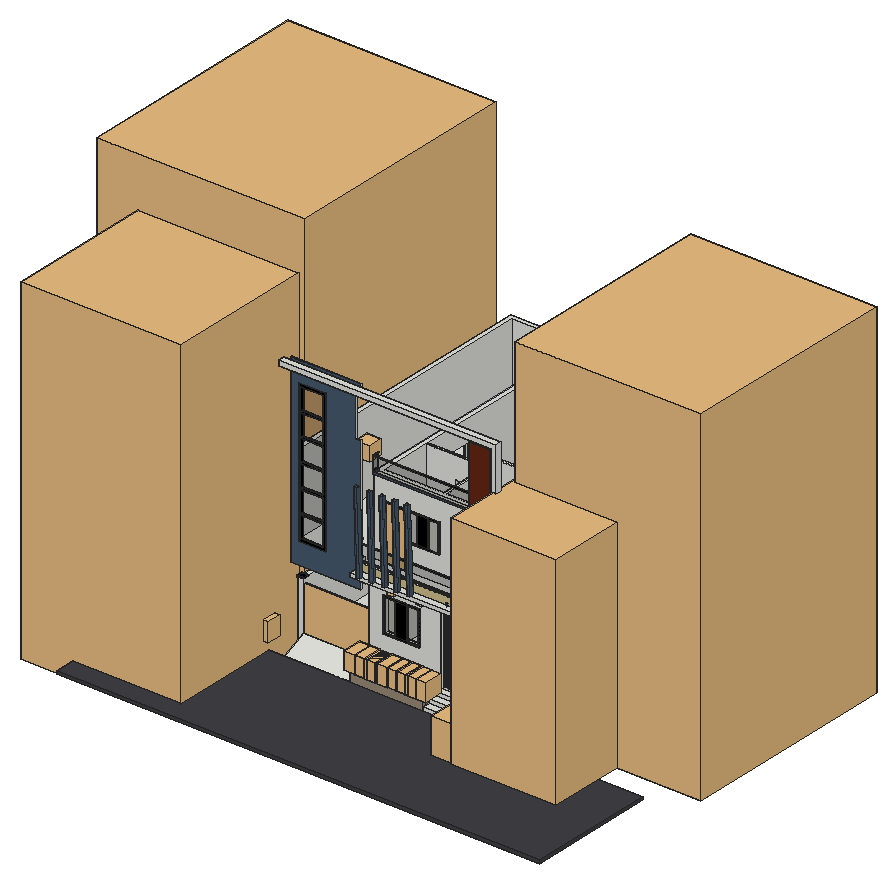
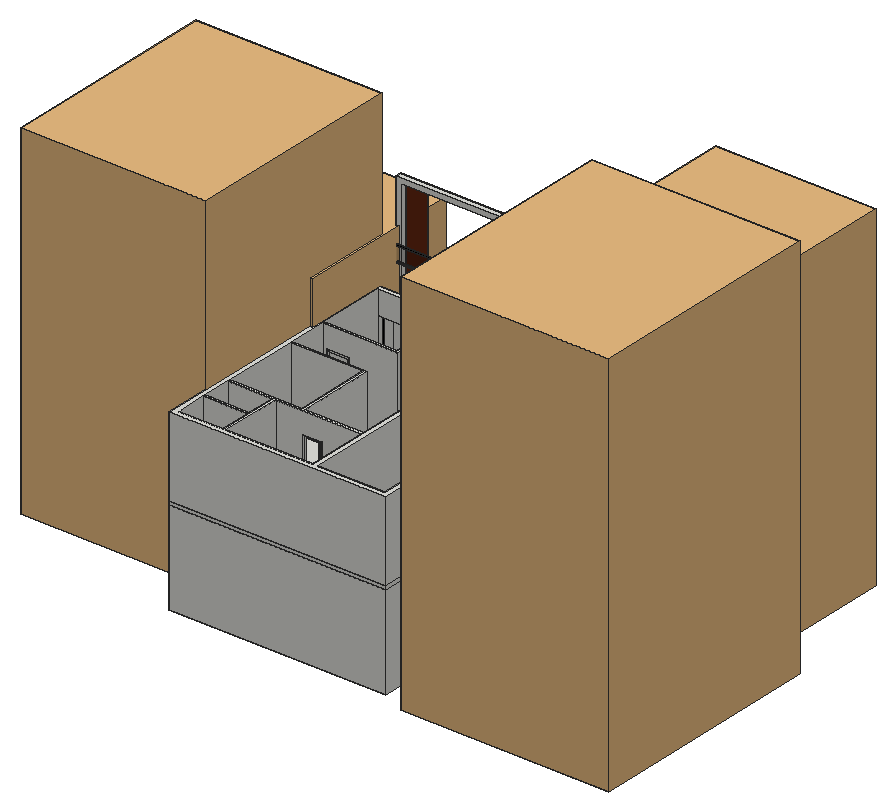
# SketchUp Ruby script. Lengths in inches.
U = 1.inch
M = Sketchup.active_model
def pt(a) = Geom::Point3d.new(a.map { |v| v * U })
def face(e, loops, mat)
  f = e.add_face(loops[0].map { |a| pt(a) })
  loops[1..].each { |l| e.add_face(l.map { |a| pt(a) }).erase! }
  f.material = f.back_material = mat if mat
  f
end
# faces: each face lists its corners as indices into pts; further lists are holes
def faces(e, pts, list, mat = nil) = list.each { |f| face(e, (f[0].is_a?(Array) ? f : [f]).map { |l| l.map { |i| pts[i] } }, mat) }
# xy, xz, yz: faces in a plane at the given z, y or x. An outline is a flat list of corners, or four numbers for a rectangle; further outlines are holes
def ring(l) = l.size == 4 ? [[l[0], l[1]], [l[2], l[1]], [l[2], l[3]], [l[0], l[3]]] : l.each_slice(2).to_a
def flat(e, list, mat, &to3) = list.each { |f| face(e, (f[0].is_a?(Array) ? f : [f]).map { |l| ring(l).map { |u, v| to3.(u, v) } }, mat) }
def xy(e, z, list, mat = nil) = flat(e, list, mat) { |x, y| [x, y, z] }
def xz(e, y, list, mat = nil) = flat(e, list, mat) { |x, z| [x, y, z] }
def yz(e, x, list, mat = nil) = flat(e, list, mat) { |y, z| [x, y, z] }
def lines(e, pts, list) = list.each { |a, b| e.add_line(pt(pts[a]), pt(pts[b])) }
# prism: a flat outline (further loops are holes) pulled along v
def prism(e, loops, v, mat = nil)
  f = face(e, loops, mat); d = Geom::Vector3d.new(v.map { |x| x * U })
  f.pushpull(f.normal.samedirection?(d) ? d.length : -d.length)
end
def box(e, o, s, mat = nil) = prism(e, [[o, [o[0] + s[0], o[1], o[2]], [o[0] + s[0], o[1] + s[1], o[2]], [o[0], o[1] + s[1], o[2]]]], [0, 0, s[2]], mat)
def at(x, y, z, deg = 0) = Geom::Transformation.translation(pt([x, y, z])) * Geom::Transformation.rotation(ORIGIN, Z_AXIS, deg.degrees)
def axes(o, x, y, z) = Geom::Transformation.new([*x, 0, *y, 0, *z, 0, *pt(o).to_a, 1])
def part(name) = M.definitions.add(name)
# library, detail: a bought-in or finely detailed component or shape, given as its bounding box
def library(name, o, s) = part(name).tap { |d| box(d.entities, o, s) }
def detail(e, o, s) = box(e.add_group.entities, o, s)
def put(e, d, t, mat = nil) = e.add_instance(d, t).tap { |i| i.material = mat if mat }
def group(e, t, mat = nil) = e.add_group.tap { |g| g.transformation = t; g.material = mat if mat }.entities
root = M.entities
M.materials.add("Asphalt Black 15-01 100cm").color = [65, 65, 69]
M.materials.add("GLass").color = [0, 0, 0]
M.materials["GLass"].alpha = 0.1
M.materials.add("Wall Paint Bumpy 01 Ochre 100cm").color = [152, 138, 118]
M.materials.add("Wall Paint Fine Grain 01 Yellow 100cm").color = [207, 190, 139]
M.materials.add("Wall Paint Simple Reflective").color = [70, 89, 109]
M.materials.add("Wood Dark 02 100cm").color = [99, 39, 19]
M.materials.add("metal").color = [0, 0, 0]
c1 = library("Tilia x europaea Pallida 007",[-304.07,-262.58,-28.16],[578.03,543.87,878])
c2 = part("Group\#50")
prism(c2.entities,[[[0,0,1.08],[0,0.04,0.8],[0,0.14,0.54],[0,0.32,0.32],[0,0.54,0.14],[0,0.8,0.04],[0,1.08,0],[0,1.36,0.04],[0,1.62,0.14],[0,1.84,0.3125],[0,1.84,1.84],[0,1.62,2.01],[0,1.36,2.12],[0,1.08,2.16],[0,0.8,2.12],[0,0.54,2.01],[0,0.32,1.84],[0,0.14,1.62],[0,0.04,1.36]]],[-101.4375,0,0])
c3 = library("Car 033",[-43.24,-98.19,-1.29],[86.48,201.64,57.79])
c4 = library("Schefflera arboricola 001",[-25.43,-22.82,-0.1],[47.76,45.73,64.24])
c5 = library("gate 134k",[0,0.67,0],[137.24,3.27,101.3])
c6 = library("Dome Light",[-12,-12,0],[24,24,12])
c7 = library("Omni Light\#2",[-12,-12,-12],[24,24,24])
c8 = library("Spot Light\#20",[-5.1,-5.1,-11.05],[10.2,10.2,11.05])
c9 = library("Spot Light\#21",[-5.1,-5.1,-11.05],[10.2,10.2,11.05])
c10 = library("Spot Light\#22",[-5.1,-5.1,-11.05],[10.2,10.2,11.05])
c11 = library("Spot Light\#23",[-5.1,-5.1,-11.05],[10.2,10.2,11.05])
c12 = library("Spot Light\#25",[-5.1,-5.1,-11.05],[10.2,10.2,11.05])
c13 = library("Spot Light\#24",[-5.1,-5.1,-11.05],[10.2,10.2,11.05])
c14 = library("Door 01",[-21.26,-2.6,0],[42.52,9.29,84.25])
c15 = library("Omni Light",[-12,-12,-12],[24,24,24])
put(root,c1,axes([25.28,470.38,-7.51],[0.59815,0,0],[0,0.73,0],[0,0,0.7332]))
put(root,c1,axes([52.75,315.37,-10.19],[0.4615,0,0],[0,1.07,0],[0,0,0.63803]))
g1 = group(root,at(197.75,0,0),"Asphalt Black 15-01 100cm")
box(g1,[-197.75,0,-5],[801.4375,215.125,5],"Asphalt Black 15-01 100cm")
g2 = group(root,at(436.25,190.68,5.33))
box(g2,[0,23.79,-6],[110.4375,39.41,6])
g3 = group(root,at(206.75,214.47,17.33))
prism(g3,[[[0,0,-17.33],[0,39.41,0],[0,39.41,-17.33]]],[108,0,0])
g4 = group(root,at(196.75,251.125,0))
g5 = group(g4,at(143.5,2.76,63.56))
xy(g5,0,[[0,-1.84,60,0]],"metal")
xy(g5,57.78,[[0,-1.84,60,0]],"metal")
xz(g5,-1.84,[[[0,0,60,57.78],[2,1.93,20,55.85],[42.01,1.93,58,55.85]]],"metal")
xz(g5,0,[[[0,0,60,57.78],[2,1.93,58,55.85]]],"metal")
yz(g5,0,[[-1.84,0,0,57.78]],"metal")
yz(g5,2,[[-1.84,1.93,0,55.85]],"metal")
yz(g5,58,[[-1.84,1.93,0,55.85]],"metal")
yz(g5,60,[[-1.84,0,0,57.78]],"metal")
g6 = group(g5,at(2,-1.84,1.93),"GLass")
box(g6,[0,0,0],[18,0.65,53.93])
g7 = group(g5,at(22,-1.84,1.93))
box(g7,[0,0,0],[18,0.65,53.93],"GLass")
g8 = group(g5,at(42.01,-1.84,1.93))
box(g8,[0,0,0],[15.99,0.65,53.93],"GLass")
g9 = group(g4,at(1,2.76,0))
xy(g9,0,[[0,0,360,441.24]])
xy(g9,17.33,[[9,0,117,0,117,8.27,119.6875,8.27,119.6875,146.83,128.6875,146.83,128.6875,99.83,178.5,99.83,178.5,96.52,128.6875,96.52,128.6875,8.27,226.5,8.27,226.5,126.31,351,126.31,351,191.39,226.5,191.39,226.5,283.85,231,283.85,231,194.7,351,194.7,351,323.76,343.72,323.76,343.72,327.07,351,327.07,351,376.71,277.1875,376.71,277.1875,327.07,309.34,327.07,309.34,323.76,226.5,323.76,226.5,327.07,272.6875,327.07,272.6875,393.16,277.1875,393.16,277.1875,380.02,351,380.02,351,432.97,277.1875,432.97,277.1875,424.97,272.6875,424.97,272.6875,432.97,128.6875,432.97,128.6875,327.07,192.375,327.07,192.375,323.76,128.6875,323.76,128.6875,214.77,119.6875,214.77,119.6875,432.97,9,432.97],[238.5,0,349.3,0,349.3,8.27,351,8.27,351,123,231,123,231,8.27,238.5,8.27]])
xy(g9,63.56,[[142.5,0,202.5,8.27]])
xy(g9,98.22,[[0,0,9,34.79]])
xy(g9,120,[[119.6875,146.83,128.6875,214.77],[226.5,283.85,231,323.76],[192.375,323.76,226.5,327.07],[309.34,323.76,343.72,327.07],[272.6875,393.16,277.1875,424.97]])
xy(g9,121.33,[[142.5,0,202.5,8.27]])
xy(g9,151.67,[[238.5,0,349.3,8.27]])
xy(g9,156,[[[117,0,360,0,360,441.24,0,441.24,0,34.79,9,34.79,9,432.97,119.6875,432.97,119.6875,8.27,117,8.27],[128.6875,8.27,128.6875,96.52,178.5,96.52,178.5,99.83,128.6875,99.83,128.6875,323.76,226.5,323.76,226.5,191.39,351,191.39,351,126.31,226.5,126.31,226.5,8.27],[231,194.7,351,323.76],[128.6875,327.07,272.6875,432.97],[231,8.27,351,123],[277.1875,380.02,351,432.97],[277.1875,327.07,351,376.71]]])
xz(g9,0,[[[0,0,360,0,360,156,117,156,117,17.33,9,17.33,9,98.22,0,98.22],[238.5,17.33,349.3,151.67],[142.5,63.56,202.5,121.33]]])
xz(g9,8.27,[[117,17.33,119.6875,156],[[128.6875,17.33,226.5,156],[142.5,63.56,202.5,121.33]],[231,17.33,231,156,351,156,351,17.33,349.3,17.33,349.3,151.67,238.5,151.67,238.5,17.33]])
xz(g9,34.79,[[0,98.22,9,156]])
xz(g9,96.52,[[128.6875,17.33,178.5,156]])
xz(g9,99.83,[[128.6875,17.33,178.5,156]])
xz(g9,123,[[231,17.33,351,156]])
xz(g9,126.31,[[226.5,17.33,351,156]])
xz(g9,146.83,[[119.6875,17.33,128.6875,120]])
xz(g9,191.39,[[226.5,17.33,351,156]])
xz(g9,194.7,[[231,17.33,351,156]])
xz(g9,214.77,[[119.6875,17.33,128.6875,120]])
xz(g9,283.85,[[226.5,17.33,231,120]])
xz(g9,323.76,[[128.6875,17.33,192.375,17.33,192.375,120,226.5,120,226.5,156,128.6875,156],[226.5,17.33,309.34,17.33,309.34,120,343.72,120,343.72,17.33,351,17.33,351,156,231,156,231,120,226.5,120]])
xz(g9,327.07,[[128.6875,17.33,128.6875,156,272.6875,156,272.6875,17.33,226.5,17.33,226.5,120,192.375,120,192.375,17.33],[277.1875,17.33,277.1875,156,351,156,351,17.33,343.72,17.33,343.72,120,309.34,120,309.34,17.33]])
xz(g9,376.71,[[277.1875,17.33,351,156]])
xz(g9,380.02,[[277.1875,17.33,351,156]])
xz(g9,393.16,[[272.6875,17.33,277.1875,120]])
xz(g9,424.97,[[272.6875,17.33,277.1875,120]])
xz(g9,432.97,[[9,17.33,119.6875,156],[128.6875,17.33,272.6875,156],[277.1875,17.33,351,156]])
xz(g9,441.24,[[0,0,360,156]])
yz(g9,0,[[0,0,0,98.22,34.79,98.22,34.79,156,441.24,156,441.24,0]])
yz(g9,9,[[0,17.33,432.97,17.33,432.97,156,34.79,156,34.79,98.22,0,98.22]])
yz(g9,117,[[0,17.33,8.27,156]])
yz(g9,119.6875,[[8.27,17.33,8.27,156,432.97,156,432.97,17.33,214.77,17.33,214.77,120,146.83,120,146.83,17.33]])
yz(g9,128.6875,[[8.27,17.33,96.52,156],[99.83,17.33,146.83,17.33,146.83,120,214.77,120,214.77,17.33,323.76,17.33,323.76,156,99.83,156],[327.07,17.33,432.97,156]])
yz(g9,142.5,[[0,63.56,8.27,121.33]])
yz(g9,178.5,[[96.52,17.33,99.83,156]])
yz(g9,192.375,[[323.76,17.33,327.07,120]])
yz(g9,202.5,[[0,63.56,8.27,121.33]])
yz(g9,226.5,[[8.27,17.33,126.31,156],[191.39,17.33,191.39,156,323.76,156,323.76,120,283.85,120,283.85,17.33],[323.76,17.33,327.07,120]])
yz(g9,231,[[8.27,17.33,123,156],[194.7,17.33,283.85,17.33,283.85,120,323.76,120,323.76,156,194.7,156]])
yz(g9,238.5,[[0,17.33,8.27,151.67]])
yz(g9,272.6875,[[327.07,17.33,327.07,156,432.97,156,432.97,17.33,424.97,17.33,424.97,120,393.16,120,393.16,17.33]])
yz(g9,277.1875,[[327.07,17.33,376.71,156],[380.02,17.33,393.16,17.33,393.16,120,424.97,120,424.97,17.33,432.97,17.33,432.97,156,380.02,156]])
yz(g9,309.34,[[323.76,17.33,327.07,120]])
yz(g9,343.72,[[323.76,17.33,327.07,120]])
yz(g9,349.3,[[0,17.33,8.27,151.67]])
yz(g9,351,[[8.27,17.33,123,156],[126.31,17.33,191.39,156],[194.7,17.33,323.76,156],[327.07,17.33,376.71,156],[380.02,17.33,432.97,156]])
yz(g9,360,[[0,0,441.24,156]])
g10 = group(g9,at(238.5,0,17.33))
xy(g10,0,[[0,-1.839,110.803,0]])
xy(g10,4.333,[[4.5,-1.839,106.303,0]])
xy(g10,130,[[4.5,-1.839,106.303,0]])
xy(g10,134.333,[[0,-1.839,110.803,0]])
xz(g10,-1.839,[[[0,0,110.803,134.333],[4.5,4.333,106.303,130]]])
xz(g10,0,[[[0,0,110.803,134.333],[4.5,4.333,106.303,130]]])
yz(g10,0,[[-1.839,0,0,134.333]])
yz(g10,4.5,[[-1.839,4.333,0,130]])
yz(g10,106.303,[[-1.839,4.333,-1.839,125.734,-1.802,125.455,-1.694,125.195,-1.523,124.972,-1.299,124.801,-1.039,124.693,-0.76,124.656,-0.481,124.693,-0.221,124.801,0,124.97,0,4.333],[0,124.97,0,126.498,0.002,126.497,0.174,126.273,0.281,126.013,0.318,125.734,0.281,125.455,0.174,125.195,0.002,124.972],[-1.839,125.734,-1.839,130,0,130,0,126.498,-0.221,126.668,-0.481,126.776,-0.76,126.8125,-1.039,126.776,-1.299,126.668,-1.523,126.497,-1.694,126.273,-1.802,126.013]])
yz(g10,110.803,[[-1.839,0,0,134.333]])
g11 = group(g10,at(4.5,-1.84,126.39),"metal")
box(g11,[-5.5,-0.92,0],[112.8,0.92,7.95])
put(g10,c2,at(106.3,-1.84,124.66),"metal")
put(g10,c2,at(106.3,-1.84,121.96),"metal")
put(g10,c2,at(106.3,-1.84,119.26),"metal")
put(g10,c2,at(106.3,-1.84,116.5625),"metal")
put(g10,c2,at(106.3,-1.84,113.86),"metal")
put(g10,c2,at(106.3,-1.84,111.17),"metal")
put(g10,c2,at(106.3,-1.84,108.47),"metal")
put(g10,c2,at(106.3,-1.84,105.77),"metal")
put(g10,c2,at(106.3,-1.84,103.07),"metal")
put(g10,c2,at(106.3,-1.84,100.375),"metal")
put(g10,c2,at(106.3,-1.84,97.68),"metal")
put(g10,c2,at(106.3,-1.84,94.98),"metal")
put(g10,c2,at(106.3,-1.84,92.28),"metal")
put(g10,c2,at(106.3,-1.84,89.58),"metal")
put(g10,c2,at(106.3,-1.84,86.89),"metal")
put(g10,c2,at(106.3,-1.84,84.1875),"metal")
put(g10,c2,at(106.3,-1.84,81.49),"metal")
put(g10,c2,at(106.3,-1.84,78.79),"metal")
put(g10,c2,at(106.3,-1.84,76.1),"metal")
put(g10,c2,at(106.3,-1.84,73.4),"metal")
put(g10,c2,at(106.3,-1.84,70.7),"metal")
put(g10,c2,at(106.3,-1.84,68),"metal")
put(g10,c2,at(106.3,-1.84,65.3),"metal")
put(g10,c2,at(106.3,-1.84,62.61),"metal")
put(g10,c2,at(106.3,-1.84,59.91),"metal")
put(g10,c2,at(106.3,-1.84,57.21),"metal")
put(g10,c2,at(106.3,-1.84,54.51),"metal")
put(g10,c2,at(106.3,-1.84,51.82),"metal")
put(g10,c2,at(106.3,-1.84,49.12),"metal")
put(g10,c2,at(106.3,-1.84,46.42),"metal")
put(g10,c2,at(106.3,-1.84,43.72),"metal")
put(g10,c2,at(106.3,-1.84,41.02),"metal")
put(g10,c2,at(106.3,-1.84,38.33),"metal")
put(g10,c2,at(106.3,-1.84,35.63),"metal")
put(g10,c2,at(106.3,-1.84,32.93),"metal")
put(g10,c2,at(106.3,-1.84,30.23),"metal")
put(g10,c2,at(106.3,-1.84,27.54),"metal")
put(g10,c2,at(106.3,-1.84,24.84),"metal")
put(g10,c2,at(106.3,-1.84,22.14),"metal")
put(g10,c2,at(106.3,-1.84,19.44),"metal")
put(g10,c2,at(106.3,-1.84,16.74),"metal")
put(g10,c2,at(106.3,-1.84,14.05),"metal")
put(g10,c2,at(106.3,-1.84,11.35),"metal")
put(g10,c2,at(106.3,-1.84,8.65),"metal")
put(g10,c2,at(106.3,-1.84,5.95),"metal")
put(g10,c2,at(106.3,-1.84,3.26),"metal")
g12 = group(g9,at(0,0,98.22),"metal")
box(g12,[-1,-0.92,0],[11,10.11,1.93])
g13 = group(g9,at(119.6875,146.83,17.33))
prism(g13,[[[0,0,0],[0,0,102.67],[0,67.9375,102.67],[0,67.9375,0]],[[0,65.9375,2],[0,65.9375,100.67],[0,2,100.67],[0,2,2]]],[2,0,0],"metal")
g14 = group(g9,at(272.6875,393.16,17.33))
prism(g14,[[[0,0,0],[0,0,102.67],[0,31.8125,102.67],[0,31.8125,0]],[[0,29.8125,2],[0,29.8125,100.67],[0,2,100.67],[0,2,2]]],[2,0,0])
g15 = group(g9,at(192.375,323.76,17.33))
prism(g15,[[[34.125,0,0],[34.125,0,102.67],[0,0,102.67],[0,0,0]],[[2,0,2],[2,0,100.67],[32.125,0,100.67],[32.125,0,2]]],[0,2,0])
g16 = group(g9,at(309.34,323.76,17.33))
prism(g16,[[[34.375,0,0],[34.375,0,102.67],[0,0,102.67],[0,0,0]],[[32.375,0,2],[2,0,2],[2,0,100.67],[32.375,0,100.67]]],[0,2,0])
g17 = group(g9,at(226.5,283.85,17.33))
prism(g17,[[[0,0,0],[0,0,102.67],[0,39.91,102.67],[0,39.91,0]],[[0,2,100.67],[0,2,2],[0,37.91,2],[0,37.91,100.67]]],[2,0,0])
g18 = group(root,at(314.75,253.88,0),"Wall Paint Bumpy 01 Ochre 100cm")
xy(g18,0,[[0,-39.41,121.5,0]])
xy(g18,1.27,[[2.5,-34.76,119,-4.64]])
xy(g18,17.33,[[[0,-39.41,121.5,0],[2.5,-34.76,119,-4.64]]])
xz(g18,-39.41,[[0,0,121.5,17.33]])
xz(g18,-34.76,[[2.5,1.27,119,17.33]])
xz(g18,-4.64,[[2.5,1.27,119,17.33]])
xz(g18,0,[[0,0,121.5,17.33]])
yz(g18,0,[[-39.41,0,0,17.33]])
yz(g18,2.5,[[-34.76,1.27,-4.64,17.33]])
yz(g18,119,[[-34.76,1.27,-4.64,17.33]])
yz(g18,121.5,[[-39.41,0,0,17.33]])
put(root,c1,axes([720,429.8125,18.41],[0.5336,0,0],[0,0.67,0],[0,0,0.65386]))
put(root,c1,axes([644.85,260.36,11.72],[0.3023,0,0],[0,0.5092,0],[0,0,0.41606]))
put(root,c3,at(616.12,171.89,1.29,-90))
g19 = group(root,at(436.25,206.67,11.33))
box(g19,[0,20.4375,-6],[110.4375,26.77,6])
g20 = group(root,at(436.25,222.38,17.33))
box(g20,[0,17.625,-6],[110.4375,13.875,6])
put(root,c4,axes([327.23,225.76,17.28],[0.71,0,0],[0,0.71,0],[0,0,0.45]))
put(root,c4,axes([345.09,225.76,17.28],[0.71,0,0],[0,0.71,0],[0,0,0.45]))
put(root,c4,axes([365.9,225.76,17.28],[0.71,0,0],[0,0.71,0],[0,0,0.45]))
put(root,c4,axes([382.15,225.76,17.28],[0.71,0,0],[0,0.71,0],[0,0,0.45]))
put(root,c4,axes([399.21,225.76,17.28],[0.71,0,0],[0,0.71,0],[0,0,0.45]))
put(root,c4,axes([413.15,225.76,17.28],[0.71,0,0],[0,0.71,0],[0,0,0.45]))
put(root,c4,axes([429.27,225.76,17.28],[0.71,0,0],[0,0.71,0],[0,0,0.45]))
put(root,c5,axes([206.75,253.21,17.33],[0.78692,0,0],[0,1,0],[0,0,0.73]))
put(root,c6,axes([160.29,215.125,18.93],[2.3904,0,0],[0,1,0],[0,0,2.59]))
g21 = group(root,at(197.75,237.97,126.6875))
g22 = group(g21,at(0,3,35.3125))
xy(g22,-35.3125,[[0,-2,117,0]])
xy(g22,0.6875,[[13.5,-3,58.5,-2]])
xy(g22,5.1875,[[18,-3,54,0]],"metal")
xy(g22,41.14,[[18,-3,54,0]],"metal")
xy(g22,43.2,[[18,-3,54,0]],"metal")
xy(g22,78.83,[[18,-3,54,0]],"metal")
xy(g22,81.51,[[18,-3,54,0]],"metal")
xy(g22,117.2,[[18,-3,54,0]],"metal")
xy(g22,119.76,[[18,-3,54,0]],"metal")
xy(g22,155.47,[[18,-3,54,0]],"metal")
xy(g22,157.47,[[18,-3,54,0]],"metal")
xy(g22,186,[[108.07,-2,117,0]])
xy(g22,193.41,[[18,-3,54,0]],"metal")
xy(g22,195.47,[[18,-3,54,0]],"metal")
xy(g22,231.5,[[18,-3,54,0]],"metal")
xy(g22,236,[[13.5,-3,58.5,-2]])
xy(g22,261,[[108.07,-2,117,0]])
xy(g22,270,[[0,-2,117,0]])
xz(g22,-3,[[[13.5,0.6875,58.5,236],[18,195.47,54,231.5],[18,5.1875,54,41.14],[18,157.47,54,193.41],[18,119.76,54,155.47],[18,81.51,54,117.2],[18,43.2,54,78.83]]],"metal")
xz(g22,-2,[[[0,-35.3125,117,-35.3125,117,186,108.07,186,108.07,261,117,261,117,270,0,270],[13.5,0.6875,58.5,236]]],"Wall Paint Simple Reflective")
xz(g22,0,[[[0,-35.3125,0,270,117,270,117,261,108.07,261,108.07,186,117,186,117,-35.3125],[18,195.47,54,231.5],[18,5.1875,54,41.14],[18,157.47,54,193.41],[18,119.76,54,155.47],[18,81.51,54,117.2],[18,43.2,54,78.83]]])
yz(g22,0,[[-2,-35.3125,0,270]])
yz(g22,13.5,[[-3,0.6875,-2,236]])
yz(g22,18,[[-3,41.14,0,43.2],[-3,78.83,0,81.51],[-3,117.2,0,119.76],[-3,155.47,0,157.47],[-3,193.41,0,195.47]])
yz(g22,18,[[-3,5.1875,0,41.14],[-3,43.2,0,78.83],[-3,81.51,0,117.2],[-3,119.76,0,155.47],[-3,157.47,0,193.41],
  [-3,195.47,0,231.5]],"metal")
yz(g22,54,[[-3,5.1875,0,41.14],[-3,43.2,0,78.83],[-3,81.51,0,117.2],[-3,119.76,0,155.47],[-3,157.47,0,193.41],
  [-3,195.47,0,231.5]],"metal")
yz(g22,58.5,[[-3,0.6875,-2,236]])
yz(g22,108.07,[[-2,186,0,261]])
yz(g22,117,[[-2,-35.3125,0,186],[-2,261,0,270]])
g23 = group(g21,at(18,0,230.8125),"GLass")
box(g23,[0,0,0],[36,0.31,36])
g24 = group(g21,at(18,0,154.6875))
box(g24,[0,0,0],[36,0.31,36],"GLass")
g25 = group(g21,at(18,0,78.5625))
box(g25,[0,0,0],[36,0.31,36],"GLass")
g26 = group(g21,at(18,0,116.625))
box(g26,[0,0,0],[36,0.31,36],"GLass")
g27 = group(g21,at(18,0,40.5))
box(g27,[0,0,0],[36,0.31,36],"GLass")
g28 = group(g21,at(18,0,192.75))
box(g28,[0,0,0],[36,0.31,36],"GLass")
put(root,c7,at(265.24,341.92,139.8125))
put(root,c8,at(325.15,233.54,155.99))
put(root,c9,at(375.07,228.99,155.99))
put(root,c10,at(419.51,232.11,155.99))
put(root,c11,at(456.9,240.4,155.99))
put(root,c12,at(541.49,228.58,155.99))
put(root,c13,at(501.71,233.79,155.99))
g29 = group(root,at(197.75,215.125,156))
xy(g29,0,[[117,0,117,25.84,0,25.84,0,480,360,480,360,0]])
xy(g29,6,[[117,0,351,0,351,9,360,9,360,12,117,12],[121.5,16.5,355.5,16.5,355.5,49.79,360,49.79,360,480,0,480,0,25.84,121.5,25.84]])
xy(g29,19,[[117,12,360,12,360,14.84,355.5,14.84,355.5,16.5,121.5,16.5,121.5,25.84,117,25.84]])
xy(g29,48,[[355.5,14.84,360,49.79]])
xy(g29,273,[[0,0,351,9]],"Wood Dark 02 100cm")
xy(g29,282,[[0,0,360,9]])
xz(g29,0,[[117,0,360,0,360,282,0,282,0,273,351,273,351,6,117,6]])
xz(g29,9,[[351,6,351,273,0,273,0,282,360,282,360,6]])
xz(g29,12,[[117,6,360,19]],"Wall Paint Fine Grain 01 Yellow 100cm")
xz(g29,14.84,[[355.5,19,360,48]])
xz(g29,16.5,[[121.5,6,355.5,19]])
xz(g29,25.84,[[0,0,117,6],[117,6,121.5,19]])
xz(g29,49.79,[[355.5,6,360,48]])
xz(g29,480,[[0,0,360,6]])
yz(g29,0,[[25.84,0,480,6],[0,273,9,282]])
yz(g29,117,[[0,0,0,6,12,6,12,19,25.84,19,25.84,0]])
yz(g29,121.5,[[16.5,6,25.84,19]])
yz(g29,351,[[0,6,9,273]])
yz(g29,355.5,[[16.5,6,16.5,19,14.84,19,14.84,48,49.79,48,49.79,6]])
yz(g29,360,[[0,0,480,0,480,6,49.79,6,49.79,48,14.84,48,14.84,19,12,19,12,6,9,6,9,282,0,282]])
g30 = group(g29,at(118.66,13.66,19),"Wall Paint Simple Reflective")
prism(g30,[[[239.68,1.18,0],[239.68,0,0],[0,0,0],[0,10.52,0],[1.18,10.52,0],[1.18,1.18,0]]],[0,0,2],"Wall Paint Simple Reflective")
g31 = group(g29,at(118.66,13.66,21),"GLass")
prism(g31,[[[239.68,1.18,0],[239.68,0,0],[0,0,0],[0,10.52,0],[1.18,10.52,0],[1.18,1.18,0]]],[0,0,24])
g32 = group(g29,at(118.66,13.66,45),"metal")
prism(g32,[[[239.68,1.18,0],[239.68,0,0],[0,0,0],[0,10.52,0],[1.18,10.52,0],[1.18,1.18,0]]],[0,0,2],"metal")
g33 = group(g29,at(144.07,13.66,157),"Wall Paint Simple Reflective")
prism(g33,[[[214.28,1.18,0],[214.28,0,0],[0,0,0],[0,10.52,0],[1.06,10.52,0],[1.06,1.18,0]]],[0,0,2],"Wall Paint Simple Reflective")
g34 = group(g29,at(144.07,13.66,159),"GLass")
prism(g34,[[[214.28,1.18,0],[214.28,0,0],[0,0,0],[0,10.52,0],[1.06,10.52,0],[1.06,1.18,0]]],[0,0,24],"GLass")
g35 = group(g29,at(144.07,13.66,183),"metal")
prism(g35,[[[214.28,1.18,0],[214.28,0,0],[0,0,0],[0,10.52,0],[1.06,10.52,0],[1.06,1.18,0]]],[0,0,2],"metal")
g36 = group(root,at(409.26,214.83,160.86),"Wall Paint Simple Reflective")
prism(g36,[[[0,5.07,0],[5.89,5.07,0],[5.89,0.08,-0.19],[0,0.08,-0.19]]],[0,-5.25,137.81],"Wall Paint Simple Reflective")
g37 = group(root,at(389.31,213.63,161.14),"Wall Paint Simple Reflective")
prism(g37,[[[0,5.07,0],[5.89,5.07,0],[5.89,0.08,-0.19],[0,0.08,-0.19]]],[0,-5.25,137.81],"Wall Paint Simple Reflective")
g38 = group(root,at(369.36,212.4375,161.43),"Wall Paint Simple Reflective")
prism(g38,[[[0,5.07,0],[5.89,5.07,0],[5.89,0.08,-0.19],[0,0.08,-0.19]]],[0,-5.25,137.81],"Wall Paint Simple Reflective")
g39 = group(root,at(349.41,211.25,161.71),"Wall Paint Simple Reflective")
prism(g39,[[[0,5.07,0],[5.89,5.07,0],[5.89,0.08,-0.19],[0,0.08,-0.19]]],[0,-5.25,137.81],"Wall Paint Simple Reflective")
g40 = group(root,at(329.46,210.05,162),"Wall Paint Simple Reflective")
prism(g40,[[[0,5.07,0],[5.89,5.07,0],[5.89,0.08,-0.19],[0,0.08,-0.19]]],[0,-5.25,137.81],"Wall Paint Simple Reflective")
g41 = group(root,at(196.75,262.23,162))
g42 = group(g41,at(173.44,2.6875,43.44))
xy(g42,0,[[0,-1.79,54.06,0]],"metal")
xy(g42,48.89,[[0,-1.79,54.06,0]],"metal")
xz(g42,-1.79,[[[0,0,54.06,48.89],[1.8,1.63,18.02,47.26],[37.86,1.63,52.26,47.26]]],"metal")
xz(g42,0,[[[0,0,54.06,48.89],[1.8,1.63,52.26,47.26]]],"metal")
yz(g42,0,[[-1.79,0,0,48.89]],"metal")
yz(g42,1.8,[[-1.79,1.63,0,47.26]],"metal")
yz(g42,52.26,[[-1.79,1.63,0,47.26]],"metal")
yz(g42,54.06,[[-1.79,0,0,48.89]],"metal")
g43 = group(g42,at(1.8,-1.79,1.63))
box(g43,[0,0,0],[16.22,0.64,45.63],"GLass")
g44 = group(g42,at(19.82,-1.79,1.63))
box(g44,[0,0,0],[16.22,0.64,45.63],"GLass")
g45 = group(g42,at(37.86,-1.79,1.63))
box(g45,[0,0,0],[14.4,0.64,45.63],"GLass")
g46 = group(g41,at(1,2.6875,0))
xy(g46,0,[[0,-23.95,0,430.21,360,430.21,360,0,289.3,0,289.3,8.07,351,8.07,351,119.92,343.6,119.92,343.6,123.15,351,123.15,351,186.6,226.5,186.6,226.5,279.85,231,279.85,231,189.83,351,189.83,351,315.66,343.72,315.66,343.72,318.89,351,318.89,351,367.29,277.1875,367.29,277.1875,318.89,303.47,318.89,303.47,315.66,226.5,315.66,226.5,318.89,272.6875,318.89,272.6875,374.52,277.1875,374.52,277.1875,370.52,351,370.52,351,422.14,277.1875,422.14,277.1875,414.34,272.6875,414.34,272.6875,422.14,128.6875,422.14,128.6875,318.89,195,318.89,195,315.66,128.6875,315.66,128.6875,186.18,119.6875,186.18,119.6875,422.14,9,422.14,9,-23.95],[117,0,117,8.07,119.6875,8.07,119.6875,143.16,128.6875,143.16,128.6875,97.33,178.5,97.33,178.5,94.11,128.6875,94.11,128.6875,8.07,136.5,8.07,136.5,0],[172.5,0,172.5,8.07,226.5,8.07,226.5,123.15,307.6,123.15,307.6,119.92,231,119.92,231,8.07,253.3,8.07,253.3,0]])
xy(g46,43.44,[[172.5,0,226.5,8.07],[289.3,0,349.3,8.07]])
xy(g46,92.33,[[136.5,0,226.5,8.07],[253.3,0,349.3,8.07]])
xy(g46,96,[[178.5,94.11,226.5,97.33],[307.6,119.92,343.6,123.15],[119.6875,143.16,128.6875,186.18],[226.5,279.85,231,315.66],[195,315.66,226.5,318.89],
  [303.47,315.66,343.72,318.89],[272.6875,374.52,277.1875,414.34]])
xy(g46,132,[[[0,-23.95,9,-23.95,9,422.14,119.6875,422.14,119.6875,8.07,117,8.07,117,0,360,0,360,430.21,0,430.21],[128.6875,97.33,128.6875,315.66,226.5,315.66,226.5,186.6,351,186.6,351,123.15,226.5,123.15,226.5,97.33],[231,189.83,351,315.66],[128.6875,318.89,272.6875,422.14],[231,8.07,351,119.92],[128.6875,8.07,226.5,94.11],[277.1875,370.52,351,422.14],[277.1875,318.89,351,367.29]]])
xz(g46,-23.95,[[0,0,9,132]])
xz(g46,0,[[117,0,136.5,0,136.5,92.33,226.5,92.33,226.5,43.44,172.5,43.44,172.5,0,253.3,0,253.3,92.33,349.3,92.33,349.3,43.44,289.3,43.44,289.3,0,360,0,360,132,117,132],[172.5,43.44,226.5,92.33],[289.3,43.44,349.3,92.33]])
xz(g46,8.07,[[117,0,119.6875,132],[128.6875,0,128.6875,132,226.5,132,226.5,92.33,136.5,92.33,136.5,0],[172.5,0,226.5,43.44],[231,0,231,132,351,132,351,0,289.3,0,289.3,43.44,349.3,43.44,349.3,92.33,253.3,92.33,253.3,0]])
xz(g46,94.11,[[128.6875,0,178.5,0,178.5,96,226.5,96,226.5,132,128.6875,132]])
xz(g46,97.33,[[128.6875,0,128.6875,132,226.5,132,226.5,96,178.5,96,178.5,0]])
xz(g46,119.92,[[231,0,307.6,0,307.6,96,343.6,96,343.6,0,351,0,351,132,231,132]])
xz(g46,123.15,[[226.5,0,226.5,132,351,132,351,0,343.6,0,343.6,96,307.6,96,307.6,0]])
xz(g46,143.16,[[119.6875,0,128.6875,96]])
xz(g46,186.18,[[119.6875,0,128.6875,96]])
xz(g46,186.6,[[226.5,0,351,132]])
xz(g46,189.83,[[231,0,351,132]])
xz(g46,279.85,[[226.5,0,231,96]])
xz(g46,315.66,[[128.6875,0,195,0,195,96,226.5,96,226.5,132,128.6875,132],[226.5,0,303.47,0,303.47,96,343.72,96,343.72,0,351,0,351,132,231,132,231,96,226.5,96]])
xz(g46,318.89,[[128.6875,0,128.6875,132,272.6875,132,272.6875,0,226.5,0,226.5,96,195,96,195,0],[277.1875,0,277.1875,132,351,132,351,0,343.72,0,343.72,96,303.47,96,303.47,0]])
xz(g46,367.29,[[277.1875,0,351,132]])
xz(g46,370.52,[[277.1875,0,351,132]])
xz(g46,374.52,[[272.6875,0,277.1875,96]])
xz(g46,414.34,[[272.6875,0,277.1875,96]])
xz(g46,422.14,[[9,0,119.6875,132],[128.6875,0,272.6875,132],[277.1875,0,351,132]])
xz(g46,430.21,[[0,0,360,132]])
yz(g46,0,[[-23.95,0,430.21,132]])
yz(g46,9,[[-23.95,0,422.14,132]])
yz(g46,117,[[0,0,8.07,132]])
yz(g46,119.6875,[[8.07,0,8.07,132,422.14,132,422.14,0,186.18,0,186.18,96,143.16,96,143.16,0]])
yz(g46,128.6875,[[8.07,0,94.11,132],[97.33,0,143.16,0,143.16,96,186.18,96,186.18,0,315.66,0,315.66,132,97.33,132],[318.89,0,422.14,132]])
yz(g46,136.5,[[0,0,8.07,92.33]])
yz(g46,172.5,[[0,0,8.07,43.44]])
yz(g46,178.5,[[94.11,0,97.33,96]])
yz(g46,195,[[315.66,0,318.89,96]])
yz(g46,226.5,[[8.07,0,8.07,43.44,0,43.44,0,92.33,8.07,92.33,8.07,132,94.11,132,94.11,96,97.33,96,97.33,132,123.15,132,123.15,0],[186.6,0,186.6,132,315.66,132,315.66,96,279.85,96,279.85,0],[315.66,0,318.89,96]])
yz(g46,231,[[8.07,0,119.92,132],[189.83,0,279.85,0,279.85,96,315.66,96,315.66,132,189.83,132]])
yz(g46,253.3,[[0,0,8.07,92.33]])
yz(g46,272.6875,[[318.89,0,318.89,132,422.14,132,422.14,0,414.34,0,414.34,96,374.52,96,374.52,0]])
yz(g46,277.1875,[[318.89,0,367.29,132],[370.52,0,374.52,0,374.52,96,414.34,96,414.34,0,422.14,0,422.14,132,370.52,132]])
yz(g46,289.3,[[0,0,8.07,43.44]])
yz(g46,303.47,[[315.66,0,318.89,96]])
yz(g46,307.6,[[119.92,0,123.15,96]])
yz(g46,343.6,[[119.92,0,123.15,96]])
yz(g46,343.72,[[315.66,0,318.89,96]])
yz(g46,349.3,[[0,43.44,8.07,92.33]])
yz(g46,351,[[8.07,0,119.92,132],[123.15,0,186.6,132],[189.83,0,315.66,132],[318.89,0,367.29,132],[370.52,0,422.14,132]])
yz(g46,360,[[0,0,430.21,132]])
g47 = group(g46,at(136.5,0,0))
prism(g47,[[[0,-1.79,92.33],[0,-1.79,0],[36,-1.79,0],[36,-1.79,92.33]],[[2,-1.79,90.33],[34,-1.79,90.33],[34,-1.79,2],[2,-1.79,2]]],[0,3.59,0],"metal")
g48 = group(g46,at(253.3,0,0))
prism(g48,[[[0,1.79,0],[0,1.79,92.33],[36,1.79,92.33],[36,1.79,0]],[[34,1.79,2],[34,1.79,90.33],[2,1.79,90.33],[2,1.79,2]]],[0,-3.59,0],"metal")
g49 = group(g46,at(272.6875,374.52,0))
prism(g49,[[[0,0,0],[0,0,96],[0,39.82,96],[0,39.82,0]],[[0,2,94],[0,2,2],[0,37.82,2],[0,37.82,94]]],[2,0,0])
g50 = group(g46,at(303.47,315.66,0))
prism(g50,[[[40.25,0,0],[40.25,0,96],[0,0,96],[0,0,0]],[[2,0,2],[2,0,94],[38.25,0,94],[38.25,0,2]]],[0,2,0])
g51 = group(g46,at(195,315.66,0))
prism(g51,[[[31.5,0,0],[31.5,0,96],[0,0,96],[0,0,0]],[[2,0,2],[2,0,94],[29.5,0,94],[29.5,0,2]]],[0,2,0])
g52 = group(g46,at(226.5,279.85,0))
prism(g52,[[[0,0,0],[0,0,96],[0,35.8125,96],[0,35.8125,0]],[[0,2,2],[0,33.8125,2],[0,33.8125,94],[0,2,94]]],[2,0,0])
g53 = group(g46,at(119.6875,143.16,0))
prism(g53,[[[0,0,0],[0,0,96],[0,43.02,96],[0,43.02,0]],[[0,41.02,94],[0,2,94],[0,2,2],[0,41.02,2]]],[2,0,0])
g54 = group(g46,at(307.6,123.15,0))
prism(g54,[[[0,0,0],[0,0,96],[36,0,96],[36,0,0]],[[2,0,94],[2,0,2],[34,0,2],[34,0,94]]],[0,-2,0])
g55 = group(g41,at(290.3,2.6875,43.44))
xy(g55,0,[[0,-1.79,60,1.79]],"metal")
xy(g55,48.89,[[0,-1.79,60,1.79]],"metal")
xz(g55,-1.79,[[[0,0,60,48.89],[2,1.63,20,47.26],[42.01,1.63,58,47.26]]],"metal")
xz(g55,1.79,[[[0,0,60,48.89],[2,1.63,58,47.26]]],"metal")
yz(g55,0,[[-1.79,0,1.79,48.89]],"metal")
yz(g55,2,[[-1.79,1.63,1.79,47.26]],"metal")
yz(g55,58,[[-1.79,1.63,1.79,47.26]],"metal")
yz(g55,60,[[-1.79,0,1.79,48.89]],"metal")
g56 = group(g55,at(2,-1.79,1.63))
box(g56,[0,0,0],[18,0.64,45.63],"GLass")
g57 = group(g55,at(22,-1.79,1.63))
box(g57,[0,0,0],[18,0.64,45.63],"GLass")
g58 = group(g55,at(42.01,-1.79,1.63))
box(g58,[0,0,0],[15.99,0.64,45.63],"GLass")
g59 = group(root,at(512.75,215.125,162),"Wood Dark 02 100cm")
box(g59,[0,-1,0],[36,1,265],"Wood Dark 02 100cm")
put(root,c14,axes([352.42,264.13,163.81],[0.75321,0,0],[0,-0.15,0],[0,0,1.05]))
put(root,c14,axes([469.23,264.13,163.81],[0.75321,0,0],[0,-0.15,0],[0,0,1.05]))
put(root,c15,at(231.52,357.41,256.0625))
